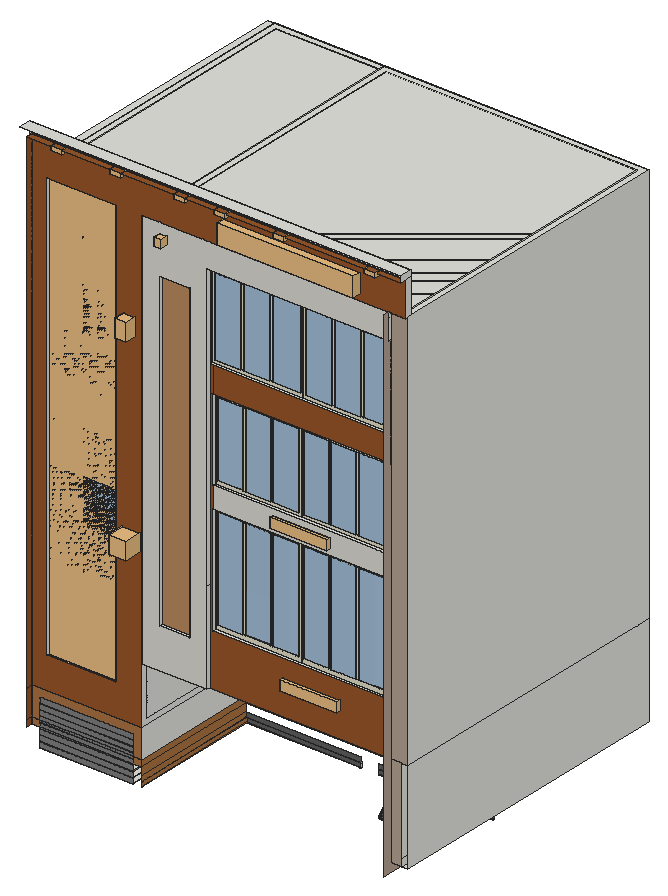
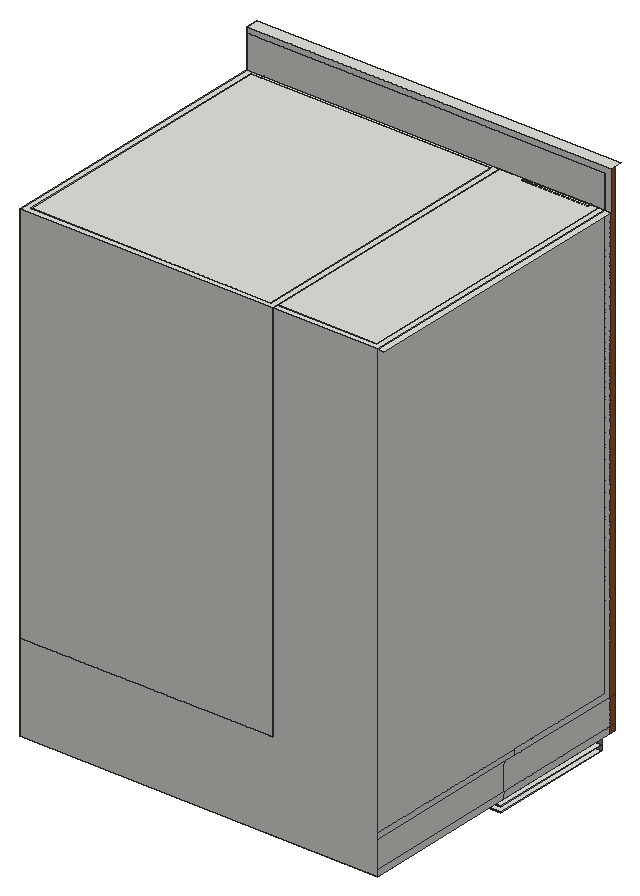
# SketchUp Ruby script. Lengths in inches.
U = 1.inch
M = Sketchup.active_model
def pt(a) = Geom::Point3d.new(a.map { |v| v * U })
def face(e, loops, mat)
  f = e.add_face(loops[0].map { |a| pt(a) })
  loops[1..].each { |l| e.add_face(l.map { |a| pt(a) }).erase! }
  f.material = f.back_material = mat if mat
  f
end
# faces: each face lists its corners as indices into pts; further lists are holes
def faces(e, pts, list, mat = nil) = list.each { |f| face(e, (f[0].is_a?(Array) ? f : [f]).map { |l| l.map { |i| pts[i] } }, mat) }
# xy, xz, yz: faces in a plane at the given z, y or x. An outline is a flat list of corners, or four numbers for a rectangle; further outlines are holes
def ring(l) = l.size == 4 ? [[l[0], l[1]], [l[2], l[1]], [l[2], l[3]], [l[0], l[3]]] : l.each_slice(2).to_a
def flat(e, list, mat, &to3) = list.each { |f| face(e, (f[0].is_a?(Array) ? f : [f]).map { |l| ring(l).map { |u, v| to3.(u, v) } }, mat) }
def xy(e, z, list, mat = nil) = flat(e, list, mat) { |x, y| [x, y, z] }
def xz(e, y, list, mat = nil) = flat(e, list, mat) { |x, z| [x, y, z] }
def yz(e, x, list, mat = nil) = flat(e, list, mat) { |y, z| [x, y, z] }
def lines(e, pts, list) = list.each { |a, b| e.add_line(pt(pts[a]), pt(pts[b])) }
# prism: a flat outline (further loops are holes) pulled along v
def prism(e, loops, v, mat = nil)
  f = face(e, loops, mat); d = Geom::Vector3d.new(v.map { |x| x * U })
  f.pushpull(f.normal.samedirection?(d) ? d.length : -d.length)
end
def box(e, o, s, mat = nil) = prism(e, [[o, [o[0] + s[0], o[1], o[2]], [o[0] + s[0], o[1] + s[1], o[2]], [o[0], o[1] + s[1], o[2]]]], [0, 0, s[2]], mat)
def at(x, y, z, deg = 0) = Geom::Transformation.translation(pt([x, y, z])) * Geom::Transformation.rotation(ORIGIN, Z_AXIS, deg.degrees)
def axes(o, x, y, z) = Geom::Transformation.new([*x, 0, *y, 0, *z, 0, *pt(o).to_a, 1])
def part(name) = M.definitions.add(name)
# library, detail: a bought-in or finely detailed component or shape, given as its bounding box
def library(name, o, s) = part(name).tap { |d| box(d.entities, o, s) }
def detail(e, o, s) = box(e.add_group.entities, o, s)
def put(e, d, t, mat = nil) = e.add_instance(d, t).tap { |i| i.material = mat if mat }
def group(e, t, mat = nil) = e.add_group.tap { |g| g.transformation = t; g.material = mat if mat }.entities
root = M.entities
M.materials.add("Glass").color = [171, 209, 242]
M.materials["Glass"].alpha = 0.09
M.materials.add("Plastic_SSS_01_White").color = [225, 221, 201]
M.materials.add("[0020_Red]").color = [234, 0, 0]
M.materials.add("[0098_DodgerBlue]").color = [162, 189, 214]
M.materials.add("[0133_Gray]").color = [96, 96, 96]
M.materials.add("[0133_Gray]1").color = [128, 128, 128]
M.materials.add("[0135_DarkGray]").color = [81, 81, 81]
M.materials.add("[Formica Speckled Grey]").color = [94, 105, 111]
M.materials.add("[Roofing Scalloped]").color = [186, 138, 96]
M.materials.add("[Terrazzo Tile Light]").color = [219, 217, 210]
M.materials.add("[Travertine Small Tile]").color = [180, 162, 145]
M.materials.add("[Wood Cherry Original]").color = [152, 86, 42]
M.materials.add("[Wood Floor]").color = [172, 116, 67]
c1 = part("Glass Door - Open Shower")
box(c1.entities,[0,0,0.95],[40,1.5,72])
c2 = library("Group\#2",[0,0,0],[96.3125,10,597])
c3 = library("SIGNAGE",[0.49,0,0],[52.61,9.87,1])
c4 = part("Window frame")
xy(c4.entities,0,[[[104.47,83.98,176.47,131.98],[106.47,85.98,174.47,129.98]],[127.47,85.98,129.47,129.98],[150.47,85.98,152.47,129.98]],"Plastic_SSS_01_White")
xy(c4.entities,2,[[[104.47,83.98,176.47,131.98],[106.47,85.98,174.47,129.98]],[127.47,85.98,129.47,129.98],[150.47,85.98,152.47,129.98]],"Plastic_SSS_01_White")
xz(c4.entities,83.98,[[104.47,0,176.47,2]],"Plastic_SSS_01_White")
xz(c4.entities,85.98,[[106.47,0,127.47,2],[127.47,0,129.47,2],[129.47,0,150.47,2],[150.47,0,152.47,2],[152.47,0,174.47,2]],"Plastic_SSS_01_White")
xz(c4.entities,129.98,[[106.47,0,127.47,2],[127.47,0,129.47,2],[129.47,0,150.47,2],[150.47,0,152.47,2],[152.47,0,174.47,2]],"Plastic_SSS_01_White")
xz(c4.entities,131.98,[[104.47,0,176.47,2]],"Plastic_SSS_01_White")
yz(c4.entities,104.47,[[83.98,0,131.98,2]],"Plastic_SSS_01_White")
yz(c4.entities,106.47,[[85.98,0,129.98,2]],"Plastic_SSS_01_White")
yz(c4.entities,127.47,[[85.98,0,129.98,2]],"Plastic_SSS_01_White")
yz(c4.entities,129.47,[[85.98,0,129.98,2]],"Plastic_SSS_01_White")
yz(c4.entities,150.47,[[85.98,0,129.98,2]],"Plastic_SSS_01_White")
yz(c4.entities,152.47,[[85.98,0,129.98,2]],"Plastic_SSS_01_White")
yz(c4.entities,174.47,[[85.98,0,129.98,2]],"Plastic_SSS_01_White")
yz(c4.entities,176.47,[[83.98,0,131.98,2]],"Plastic_SSS_01_White")
c5 = part("Window pane")
box(c5.entities,[0,0,0],[67.88,44,0.5])
c6 = part("Glazed window unit")
put(c6.entities,c4,at(-104.47,-83.98,0))
put(c6.entities,c5,at(2,2,0.7),"Glass")
c7 = part("window")
p = [[-596.28,88.12,20.39],[-668.28,88.12,20.39]]
lines(c7.entities,p,[[0,1]])
put(c7.entities,c6,axes([-668.28,88.12,20.39],[1,0,0],[0,0,1],[0,-1,0]))
c8 = library("Omni Light\#3",[-12,-12,-12],[24,24,24])
c9 = library("Omni Light\#2",[-12,-12,-12],[24,24,24])
c10 = library("Spot Light",[-5.1,-5.1,-11.05],[10.2,10.2,11.05])
c11 = library("Building Name",[0.96,0,0],[81.96,12.64,1])
c12 = library("Omni Light\#4",[-12,-12,-12],[24,24,24])
xy(root,93.95,[[21,9,150.5,192.6875]])
xy(root,94.45,[[21,9,150.5,192.6875]])
xy(root,94.7,[[347,191.6875,507.47,192.6875],[162.5,192.0625,322.97,192.6875]])
xy(root,95.2,[[347,191.6875,507.47,192.6875],[162.5,192.0625,322.97,192.6875]])
xy(root,101.1,[[346.99,191.6875,507.46,192.6875],[162.5,192.0625,322.97,192.6875]])
xy(root,101.6,[[162.5,191.6875,322.97,192.6875],[346.99,191.6875,507.45,192.6875]])
xy(root,101.82,[[21,9,150.5,192.6875]])
xy(root,102.32,[[21,9,150.5,192.6875]])
xy(root,102.5,[[[404.69,160.97,507.9,164.35,506.48,179.71,403.27,176.33],[414.3,165.74,413.36,165.77,412.49,165.95,411.73,166.27,411.15,166.72,410.78,167.26,410.65,167.86,410.76,168.47,411.12,169.06,411.69,169.57,412.43,169.99,413.3,170.28,414.23,170.41,415.17,170.39,416.04,170.21,416.8,169.88,417.38,169.43,417.75,168.89,417.88,168.29,417.77,167.68,417.41,167.1,416.85,166.58,416.1,166.17,415.23,165.88]],[414.3,165.74,415.23,165.88,416.1,166.17,416.85,166.58,417.41,167.1,417.77,167.68,417.88,168.29,417.75,168.89,417.38,169.43,416.8,169.88,416.04,170.21,415.17,170.39,414.23,170.41,413.3,170.28,412.43,169.99,411.69,169.57,411.12,169.06,410.76,168.47,410.65,167.86,410.78,167.26,411.15,166.72,411.73,166.27,412.49,165.95,413.36,165.77],[403.27,176.33,401.86,191.6875,505.0625,195.07,506.48,179.71]],"[Formica Speckled Grey]")
xy(root,109.69,[[21,9,150.5,192.6875]])
xy(root,110.19,[[21,9,150.5,192.6875]])
xy(root,117.14,[[[403.27,176.33,506.48,179.71,505.0625,195.07,401.86,191.6875],[412.3,181.1,412.125,181.12,411.95,181.125,411.67,181.18,411.39,181.22,411.24,181.27,411.07,181.31,410.84,181.41,410.59,181.49,410.46,181.57,410.32,181.63,410.14,181.77,409.93,181.9,409.85,182,409.74,182.08,409.62,182.25,409.48,182.41,409.4375,182.52,409.37,182.625,409.33,182.81,409.26,182.99,409.26,183.11,409.23,183.22,409.27,183.41,409.28,183.6,409.33,183.71,409.35,183.83,409.46,184.01,409.54,184.2,409.63,184.3,409.7,184.42,409.88,184.58,410.03,184.75,410.16,184.83,410.27,184.93,410.5,185.0625,410.71,185.2,410.87,185.27,411.01,185.35,411.28,185.4375,411.54,185.54,411.72,185.58,411.88,185.63,412.17,185.68,412.46,185.74,412.64,185.74,412.82,185.77,413.11,185.76,413.4,185.77,413.57,185.75,413.75,185.75,414.03,185.69,414.31,185.65,414.46,185.6,414.63,185.57,414.86,185.46,415.11,185.38,415.24,185.3,415.38,185.24,415.5625,185.1,415.77,184.97,415.85,184.88,415.96,184.79,416.08,184.625,416.22,184.46,416.26,184.35,416.33,184.25,416.375,184.06,416.44,183.88,416.44,183.77,416.47,183.65,416.43,183.46,416.42,183.27,416.375,183.16,416.35,183.04,416.24,182.86,416.16,182.67,416.07,182.57,416,182.46,415.82,182.3,415.67,182.125,415.54,182.04,415.43,181.94,415.2,181.8125,414.99,181.67,414.83,181.6,414.6875,181.52,414.42,181.4375,414.16,181.33,413.98,181.29,413.82,181.24,413.53,181.2,413.24,181.14,413.0625,181.13,412.88,181.1,412.59,181.11]],[412.88,181.1,413.0625,181.13,412.59,181.11],[412.125,181.12,411.67,181.18,411.95,181.125],[413.53,181.2,413.82,181.24,413.98,181.29],[411.24,181.27,410.84,181.41,411.07,181.31],
  [414.42,181.4375,414.6875,181.52,414.83,181.6],[410.46,181.57,410.14,181.77,410.32,181.63],[415.2,181.8125,415.43,181.94,415.54,182.04],[409.85,182,409.62,182.25,409.74,182.08],[415.82,182.3,416,182.46,416.07,182.57],
  [409.4375,182.52,409.33,182.81,409.37,182.625],[416.24,182.86,416.35,183.04,416.375,183.16],[409.26,183.11,409.27,183.41,409.23,183.22],[416.43,183.46,416.47,183.65,416.44,183.77],[409.33,183.71,409.46,184.01,409.35,183.83],
  [416.375,184.06,416.33,184.25,416.26,184.35],[409.63,184.3,409.88,184.58,409.7,184.42],[416.08,184.625,415.96,184.79,415.85,184.88],[410.16,184.83,410.5,185.0625,410.27,184.93],[415.5625,185.1,415.38,185.24,415.24,185.3],
  [410.87,185.27,411.28,185.4375,411.01,185.35],[414.86,185.46,414.63,185.57,414.46,185.6],[411.72,185.58,412.17,185.68,411.88,185.63],[414.03,185.69,413.75,185.75,413.57,185.75],[412.64,185.74,413.11,185.76,412.82,185.77]],"[Formica Speckled Grey]")
xy(root,117.5625,[[21,9,150.5,192.6875]])
xy(root,118.0625,[[21,9,150.5,192.6875]])
xy(root,120,[[9,9,9,201.6875,18,201.6875,18,423.6875,522.4375,423.6875,522.4375,201.6875,162.5,201.6875,162.5,9],[522.4375,13,522.4375,191.6875,162.5,191.6875,162.5,201.6875,522.4375,201.6875,522.4375,423.6875,18,423.6875,18,201.6875,9,201.6875,9,432.6875,531.4375,432.6875,531.4375,13]])
xy(root,120,[[507.4375,13,522.4375,191.6875]],"[Travertine Small Tile]")
xy(root,125.43,[[21,191.6875,150.5,192.6875]])
xy(root,125.43,[[21,9,150.5,191.6875]],"[0133_Gray]1")
xy(root,125.93,[[21,191.6875,150.5,192.6875]])
xy(root,125.93,[[21,9,150.5,191.6875]],"[0133_Gray]1")
xy(root,129,[[9,9,162.5,9,162.5,423.6875,18,423.6875,18,201.6875,9,201.6875],[162.5,191.6875,507.4375,215.6875],[507.4375,191.6875,522.4375,215.6875],[186.5,215.6875,504.4375,215.6875,504.4375,224.6875,522.4375,224.6875,522.4375,423.6875,186.5,423.6875]])
xy(root,133.3,[[21,9,150.5,192.6875]])
xy(root,133.8,[[21,9,150.5,192.6875]])
xy(root,141.18,[[21,9,150.5,192.6875]])
xy(root,141.68,[[21,9,150.5,192.6875]])
xy(root,149.05,[[21,9,150.5,192.6875]])
xy(root,149.55,[[21,9,150.5,192.6875]])
xy(root,168,[[18,9,162.5,201.6875],[9,181.6875,18,201.6875]])
xy(root,168,[[9,9,18,181.6875]],"[Wood Floor]")
xy(root,177,[[9,18,18,181.6875],[18,18,162.5,201.6875]])
xy(root,213,[[30.5,9,126,18]])
xy(root,232,[[186.5,215.6875,504.4375,224.6875]])
xy(root,249,[[162.5,9,162.5,215.6875,522.4375,215.6875,522.4375,13,254.07,13,254.07,9],[522.4375,13,531.4375,432.6875],[162.5,215.6875,162.5,432.6875,522.4375,432.6875,522.4375,423.6875,186.5,423.6875,186.5,224.6875,522.4375,224.6875,522.4375,215.6875],[186.5,224.6875,522.4375,423.6875]])
xy(root,258,[[171.5,22,522.4375,423.6875]])
xy(root,305.18,[[187.89,9,230.08,13]])
xy(root,322.125,[[259.07,13,498.4375,22]])
xy(root,474,[[259.07,13,498.4375,22]])
xy(root,504,[[259.07,13,498.4375,22]])
xy(root,618,[[259.07,13,498.4375,22],[498.4375,13,507.4375,22]])
xy(root,654,[[254.07,13,507.4375,22]])
xy(root,742.06,[[187.89,9,230.08,13]])
xy(root,774,[[254.07,9,507.4375,13],[254.07,13,507.4375,22]])
xy(root,810,[[30.5,9,30.5,18,126.5,18,126,9],[126,9,126.5,18,162.5,18,162.5,9],[162.5,9,507.4375,18],[507.4375,9,531.4375,13],[507.4375,13,507.4375,22,522.4375,22,522.4375,423.6875,171.5,423.6875,171.5,22,507.4375,22,507.4375,18,531.4375,18,531.4375,13],
  [507.4375,13,531.4375,18],[0,18,9,432.6875],[9,18,18,18,18,423.6875,162.5,423.6875,162.5,432.6875,9,432.6875],[18,18,162.5,423.6875],[162.5,18,531.4375,432.6875]])
xy(root,858,[[9,9,531.4375,18]])
xy(root,858,[[9,0,531.4375,9]],"[Wood Cherry Original]")
xy(root,866.75,[[0,0,531.4375,18]])
xz(root,9,[[21,94.45,150.5,101.82],[21,102.32,150.5,109.69],[21,110.19,150.5,117.5625],[21,118.0625,150.5,120],[21,120,150.5,125.43],
  [21,125.93,150.5,129],[21,129,150.5,133.3],[21,133.8,150.5,141.18],[21,141.68,150.5,149.05],[21,149.55,150.5,157.42]],"[0133_Gray]1")
xz(root,9,[[[162.5,249,254.07,249,254.07,774,507.4375,774,507.4375,810,162.5,810],[187.89,305.18,230.08,742.06]]],"[Terrazzo Tile Light]")
xz(root,9,[[9,168,162.5,168,162.5,810,126,810,126,213,30.5,213,30.5,810,531.4375,810,531.4375,858,9,858]],"[Wood Cherry Original]")
xz(root,9,[[9,120,21,129],[150.5,120,162.5,129],[9,129,21,129,21,157.42,150.5,157.42,150.5,129,162.5,129,162.5,168,9,168]],"[Wood Floor]")
xz(root,13,[[78.1,630.9,78.18,690.1],[78.1,690.54,124.85,690.6,78.1,690.6]])
xz(root,13,[[30.76,332.4,78.59,392.1],[78.59,332.4,125.26,392.1],[30.76,392.1,78.43,451.3],[78.43,392.1,125.18,451.3],[78.34,451.3,125.18,511],
  [30.68,451.8,77.84,511],[30.43,511.5,77.84,571.2],[78.34,511.5,125.01,571.2],[30.43,571.2,77.76,630.4],[78.26,571.2,124.93,630.4],
  [30.5,630.9,78.1,690.1],[78.18,630.9,124.93,630.9,124.93,690.6,124.85,690.6,78.1,690.54,78.1,690.1,78.18,690.1],[30.5,690.6,77.6,749.8],[78.1,690.6,124.85,690.6,124.77,750.36,78.02,750.3],[30.5,750.3,77.9375,809.5],
  [78.02,750.3,124.77,750.36,124.6875,809.5,77.9375,809.4375]],"[0098_DodgerBlue]")
xz(root,13,[[187.89,305.18,230.08,742.06]],"[Roofing Scalloped]")
xz(root,13,[[259.07,474,498.4375,504]],"[Terrazzo Tile Light]")
xz(root,13,[[507.4375,120,522.4375,249],[507.4375,249,531.4375,810]],"[Travertine Small Tile]")
xz(root,13,[[254.07,249,507.4375,249,507.4375,618,498.4375,618,498.4375,322.125,259.07,322.125,259.07,618,254.07,618],[254.07,618,259.07,654],[259.07,618,498.4375,654],[498.4375,618,507.4375,654]],"[Wood Cherry Original]")
xz(root,13.5,[[31,213.5,78.25,213.5625,78.17,272.2,30.92,272.14],[78.67,213.5,125.5,272.2],[30.92,272.7,78.67,272.76,78.59,331.9,30.84,331.84],[78.67,272.7,125.34,331.9]],"[0098_DodgerBlue]")
xz(root,17.5,[[262.4,328.54,297.31,469.78],[382.08,328.54,416.99,469.78],[420.3125,328.54,455.22,469.78],[300.63,508.75,335.54,613.25],[338.86,508.75,375.43,613.25],
  [382.08,508.75,416.99,613.25],[420.3125,508.75,455.22,613.25],[458.54,508.75,495.11,613.25],[257.6,658.94,294.67,767.62],[298.19,658.94,335.26,767.62],
  [338.79,658.94,377.61,767.62],[384.67,658.94,421.73,767.62],[425.26,658.94,462.33,767.62]],"[0098_DodgerBlue]")
xz(root,18,[[18,177,18,810,30.5,810,30.5,213,126,213,126.5,810,162.5,810,162.5,177],[30.5,213,30.5,810,126.5,810,126,213],[0,810,0,866.75,531.4375,866.75,531.4375,858,9,858,9,810],[9,810,531.4375,858]])
xz(root,22,[[[171.5,258,171.5,810,507.4375,810,507.4375,774,254.07,774,254.07,654,507.4375,654,507.4375,618,259.07,618,259.07,504,498.4375,504,498.4375,618,507.4375,618,507.4375,258],[259.07,322.125,498.4375,474]],[507.4375,258,522.4375,810]])
xz(root,181.6875,[[9,168,18,177]])
xz(root,191.6875,[[162.5,120,507.4375,129],[507.4375,120,522.4375,129],[21,125.43,150.5,125.93]])
xz(root,191.6875,[[347,95.2,507.47,95.2,507.46,101.1,346.99,101.1],[162.5,101.6,322.97,108],[346.99,101.6,507.45,101.6,507.4375,108,346.97,108]],"[0133_Gray]")
xz(root,192.0625,[[162.5,95.2,322.97,101.1]],"[0133_Gray]")
xz(root,192.6875,[[347,94.7,507.47,95.2],[346.99,101.1,507.46,101.1,507.45,101.6,346.99,101.6]])
xz(root,192.6875,[[21,93.95,150.5,94.45],[162.5,94.7,322.97,95.2],[162.5,101.1,322.97,101.6],[21,101.82,150.5,102.32],[21,109.69,150.5,110.19],
  [21,117.5625,150.5,118.0625],[21,125.43,150.5,125.93],[21,133.3,150.5,133.8],[21,141.18,150.5,141.68],[21,149.05,150.5,149.55]],"[0135_DarkGray]")
xz(root,201.6875,[[9,120,18,129],[9,129,18,168],[18,168,162.5,177]])
xz(root,215.6875,[[162.5,129,186.5,129,186.5,232,504.4375,232,504.4375,129,522.4375,129,522.4375,249,162.5,249]],"[0133_Gray]")
xz(root,224.6875,[[504.4375,129,504.4375,232,186.5,232,186.5,249,522.4375,249,522.4375,129]])
xz(root,423.6875,[[18,129,162.5,810],[186.5,129,522.4375,249],[171.5,258,522.4375,810]])
xz(root,432.6875,[[9,120,9,810,162.5,810,162.5,249,531.4375,249,531.4375,120],[162.5,249,531.4375,810]])
yz(root,9,[[9,120,201.6875,129],[201.6875,120,432.6875,129],[9,129,201.6875,168],[201.6875,129,432.6875,168],[9,168,9,858,18,858,18,177,181.6875,177,181.6875,168],
  [181.6875,168,432.6875,177],[18,177,432.6875,810]])
yz(root,9,[[0,120,9,129],[0,129,9,168],[0,168,9,858]],"[Wood Cherry Original]")
yz(root,18,[[201.6875,129,423.6875,129,423.6875,810,18,810,18,177,201.6875,177],[181.6875,168,201.6875,177]])
yz(root,21,[[9,93.95,192.6875,94.45],[9,101.82,192.6875,102.32],[9,109.69,192.6875,110.19],[9,117.5625,192.6875,118.0625],[191.6875,125.43,192.6875,125.93],
  [9,133.3,192.6875,133.8],[9,141.18,192.6875,141.68],[9,149.05,192.6875,149.55]])
yz(root,21,[[9,125.43,191.6875,125.93]],"[Wood Floor]")
yz(root,30.5,[[9,213,18,810]])
yz(root,150.5,[[191.6875,125.43,192.6875,125.93],[9,133.3,192.6875,133.8],[9,141.18,192.6875,141.68],[9,149.05,192.6875,149.55]])
yz(root,150.5,[[9,93.95,192.6875,94.45],[9,101.82,192.6875,102.32],[9,109.69,192.6875,110.19],[9,117.5625,192.6875,118.0625],[9,125.43,191.6875,125.93]],"[Wood Floor]")
yz(root,162.5,[[191.6875,120,201.6875,129],[9,129,201.6875,168],[201.6875,129,215.6875,177],[215.6875,129,423.6875,249],[9,168,201.6875,168,201.6875,177,18,177,18,249,9,249],
  [18,177,215.6875,249],[9,249,18,810],[18,249,423.6875,810],[423.6875,249,432.6875,810]])
yz(root,162.5,[[9,94.7,192.6875,95.2],[9,95.2,192.0625,101.1],[9,101.1,192.6875,101.6],[9,101.6,191.6875,108],[9,108,191.6875,120],
  [9,120,191.6875,129]],"[Wood Floor]")
yz(root,171.5,[[22,258,423.6875,810]])
yz(root,186.5,[[215.6875,129,423.6875,129,423.6875,249,224.6875,249,224.6875,232,215.6875,232]])
yz(root,187.89,[[9,305.18,13,742.06]])
yz(root,230.08,[[9,305.18,13,742.06]])
yz(root,254.07,[[9,249,13,378],[9,378,13,774],[13,654,22,774]])
yz(root,259.07,[[13,322.125,22,474],[13,504,22,618]])
yz(root,322.97,[[191.6875,94.7,192.6875,95.2],[191.6875,95.2,192.0625,101.1],[191.6875,101.1,192.6875,101.6]])
yz(root,346.99,[[191.6875,101.1,192.6875,101.6]])
yz(root,347,[[191.6875,94.7,192.6875,95.2]])
yz(root,498.4375,[[13,322.125,22,474],[13,504,22,618]])
yz(root,504.4375,[[215.6875,129,224.6875,232]])
yz(root,507.4375,[[13,618,22,654],[13,654,22,774],[9,774,13,810],[13,774,22,810]])
yz(root,507.4375,[[0.125,108,0.125,810,9,810,9,774,13,774,13,120,191.6875,120,191.6875,108]],"[Travertine Small Tile]")
yz(root,522.4375,[[13,120,191.6875,129],[13,129,215.6875,249],[215.6875,129,224.6875,249],[224.6875,129,423.6875,249],[22,258,423.6875,810]])
yz(root,531.4375,[[13,120,432.6875,249],[13,249,432.6875,810],[9,810,18,858],[0,858,18,866.75]])
p = [[416.78,122.77,113.62],[416.68,123.91,114.71],[417.55,124.2,114.47],[417.66,122.95,113.27],[418.96,108.84,99.82],[418.09,108.56,100.06],
  [418.48,124.34,114.41],[418.6,123.05,113.1875],[419.9,108.98,99.77],[419.42,124.3125,114.54],[419.53,123.09,113.375],[420.83,108.95,99.9],
  [420.29,124.13,114.84],[420.39,123.05,113.82],[421.71,108.77,100.2],[416.02,122.55,114.21],[415.93,123.5,115.11],[417.35,108.14,100.47],
  [421.05,123.8,115.31],[421.125,122.94,114.49],[422.46,108.45,100.66],[415.43,122.28,114.99],[415.37,122.98,115.66],[416.78,107.62,101.01],
  [421.63,123.36,115.89],[421.68,122.77,115.34],[423.04,108,101.25],[415.05,122,115.93],[415.01,122.4,116.3],[416.43,107.04,101.66],
  [422,122.81,116.57],[422.02,122.55,116.31],[423.41,107.46,101.92],[414.9,121.72,116.94],[414.9,121.78,117],[416.3125,106.43,102.36],
  [422.13,122.22,117.28],[423.54,106.92,102.69],[423.55,106.86,102.63],[416.42,106.1,103.33],[415.03,121.1875,117.71],[416.45,105.83,103.07],
  [413.36,165.77,102.5],[414.3,165.74,102.5],[414.3,165.74,163.8],[413.36,165.77,163.67],[415.23,165.88,102.5],[415.23,165.88,163.74],
  [412.49,165.95,102.5],[412.49,165.95,163.36],[411.73,166.27,102.5],[411.73,166.27,162.9],[416.1,166.17,102.5],[416.1,166.17,163.5],
  [416.85,166.58,102.5],[416.85,166.58,163.09],[411.15,166.72,102.5],[411.15,166.72,162.31],[417.41,167.1,102.5],[417.41,167.1,162.55],
  [410.78,167.26,102.5],[410.78,167.26,161.64],[417.77,167.68,102.5],[417.77,167.68,161.91],[410.65,167.86,102.5],[410.65,167.86,160.93],
  [417.88,168.29,102.5],[417.88,168.29,161.2],[410.76,168.47,102.5],[410.76,168.47,160.23],[417.75,168.89,102.5],[417.75,168.89,160.49],
  [411.12,169.06,102.5],[411.12,169.06,159.58],[417.38,169.43,102.5],[417.38,169.43,159.82],[411.69,169.57,102.5],[411.69,169.57,159.04],
  [416.8,169.88,102.5],[416.8,169.88,159.23],[412.43,169.99,102.5],[412.43,169.99,158.63],[416.04,170.21,102.5],[416.04,170.21,158.77],
  [413.3,170.28,102.5],[413.3,170.28,158.39],[415.17,170.39,102.5],[415.17,170.39,158.47],[414.23,170.41,102.5],[414.23,170.41,158.34],
  [401.86,191.6875,102.5],[403.27,176.33,102.5],[403.27,176.33,117.14],[401.86,191.6875,117.14],[506.48,179.71,102.5],[506.48,179.71,117.14],
  [505.0625,195.07,102.5],[505.0625,195.07,117.14],[422.02,121.61,117.98],[423.4,106.64,103.71],[423.43,106.25,103.34],[416.76,105.875,104.3],
  [415.4,120.65,118.39],[416.82,105.29,103.74],[421.66,121.02,118.625],[423.01,106.36,104.64],[423.08,105.66,103.98],[417.32,105.7,105.15],
  [415.98,120.2,118.97],[417.4,104.84,104.33],[421.09,120.5,119.17],[422.42,106.1,105.43],[422.51,105.15,104.52],[418.05,105.59,105.82],
  [416.74,119.87,119.4375],[418.15,104.51,104.79],[420.35,120.09,119.57],[421.66,105.87,106.02],[421.77,104.73,104.93],[418.91,105.55,106.26],
  [417.61,119.69,119.74],[419.03,104.33,105.1],[419.48,119.8,119.8125],[420.78,105.7,106.37],[420.9,104.44,105.17],[419.85,105.59,106.45],
  [418.55,119.67,119.87],[419.96,104.31,105.23],[416.25,138.3,127.91],[416.13,139.56,129.11],[417.0625,139.69,129.05],[417.18,138.41,127.83],
  [418,139.67,129.18],[418.11,138.45,128.02],[415.37,138.13,128.26],[415.26,139.27,129.35],[418.875,139.49,129.49],[418.98,138.41,128.46],
  [414.61,137.91,128.85],[414.52,138.86,129.76],[419.63,139.16,129.95],[419.71,138.3,129.13],[414.01,137.64,129.64],[413.95,138.34,130.3],
  [420.21,138.71,130.54],[420.27,138.13,129.98],[413.63,137.36,130.57],[413.6,137.75,130.94],[420.58,138.17,131.21],[420.61,137.9,130.95],
  [413.49,137.08,131.59],[413.48,137.14,131.65],[420.71,137.58,131.92],[422.125,122.28,117.34],[415.01,121.46,117.97],[413.61,136.55,132.36],
  [412.3,181.1,168.71],[411.39,181.22,169.34],[411.39,181.22,117.14],[411.67,181.18,117.14],[412.125,181.12,117.14],[412.3,181.1,117.14],
  [413.24,181.14,168.5625],[412.59,181.11,117.14],[413.0625,181.13,117.14],[413.24,181.14,117.14],[414.16,181.33,168.9],[413.53,181.2,117.14],
  [413.98,181.29,117.14],[414.16,181.33,117.14],[410.59,181.49,170.4],[410.59,181.49,117.14],[410.84,181.41,117.14],[411.24,181.27,117.14],
  [414.99,181.67,169.7],[414.42,181.4375,117.14],[414.83,181.6,117.14],[414.99,181.67,117.14],[409.93,181.9,171.83],[409.93,181.9,117.14],
  [410.14,181.77,117.14],[410.46,181.57,117.14],[415.67,182.125,170.91],[415.2,181.8125,117.14],[415.54,182.04,117.14],[415.67,182.125,117.14],
  [409.48,182.41,173.52],[409.48,182.41,117.14],[409.62,182.25,117.14],[409.85,182,117.14],[416.16,182.67,172.45],[415.82,182.3,117.14],
  [416.07,182.57,117.14],[416.16,182.67,117.14],[409.26,182.99,175.35],[409.26,182.99,117.14],[409.33,182.81,117.14],[409.4375,182.52,117.14],
  [416.42,183.27,174.2],[416.24,182.86,117.14],[416.375,183.16,117.14],[416.42,183.27,117.14],[409.28,183.6,177.22],[409.28,183.6,117.14],
  [409.27,183.41,117.14],[409.26,183.11,117.14],[416.44,183.88,176.07],[416.43,183.46,117.14],[416.44,183.77,117.14],[416.44,183.88,117.14],
  [409.54,184.2,178.97],[409.54,184.2,117.14],[409.46,184.01,117.14],[409.33,183.71,117.14],[416.22,184.46,177.9],[416.375,184.06,117.14],
  [416.26,184.35,117.14],[416.22,184.46,117.14],[410.03,184.75,180.51],[410.03,184.75,117.14],[409.88,184.58,117.14],[409.63,184.3,117.14],
  [415.77,184.97,179.59],[416.08,184.625,117.14],[415.85,184.88,117.14],[415.77,184.97,117.14],[410.71,185.2,181.72],[410.71,185.2,117.14],
  [410.5,185.0625,117.14],[410.16,184.83,117.14],[415.11,185.38,181.02],[415.5625,185.1,117.14],[415.24,185.3,117.14],[415.11,185.38,117.14],
  [411.54,185.54,182.52],[411.54,185.54,117.14],[411.28,185.4375,117.14],[410.87,185.27,117.14],[414.31,185.65,182.08],[414.86,185.46,117.14],
  [414.46,185.6,117.14],[414.31,185.65,117.14],[412.46,185.74,182.86],[412.46,185.74,117.14],[412.17,185.68,117.14],[411.72,185.58,117.14],
  [413.4,185.77,182.71],[413.4,185.77,117.14],[413.11,185.76,117.14],[412.64,185.74,117.14],[414.03,185.69,117.14],[413.57,185.75,117.14],
  [420.6,136.97,132.62],[421.98,122,118.35],[415.35,121.23,118.94],[413.98,136.01,133.03],[420.25,136.38,133.27],[421.6,121.72,119.29],
  [415.9,121.06,119.79],[414.56,135.56,133.62],[419.68,135.86,133.81],[421.01,121.46,120.07],[416.64,120.95,120.46],[415.32,135.23,134.08],
  [418.93,135.45,134.22],[420.25,121.23,120.66],[417.5,120.91,120.91],[416.19,135.05,134.38],[418.07,135.16,134.46],[419.37,121.06,121.01],
  [418.43,120.95,121.09],[417.13,135.03,134.51],[413.85,154.63,143.99],[414.71,154.92,143.75],[414.83,153.66,142.56],[413.95,153.49,142.9],
  [415.65,155.05,143.69],[415.77,153.77,142.47],[416.59,155.03,143.82],[416.7,153.81,142.66],[417.46,154.85,144.13],[417.56,153.77,143.1],
  [413.1,154.22,144.4],[413.1875,153.27,143.49],[418.22,154.52,144.59],[418.29,153.66,143.77],[412.6,153,144.28],[412.53,153.7,144.94],
  [418.8,154.07,145.18],[418.85,153.49,144.62],[412.22,152.72,145.21],[412.18,153.11,145.59],[419.17,153.53,145.85],[419.19,153.26,145.59],
  [412.07,152.4375,146.23],[412.07,152.5,146.29],[419.3,152.9375,146.5625],[420.71,137.64,131.98],[413.59,136.82,132.61],[412.2,151.91,147],
  [419.18,152.32,147.26],[420.5625,137.36,133],[413.93,136.59,133.59],[412.57,151.36,147.67],[418.83,151.74,147.91],[420.18,137.08,133.93],
  [414.49,136.42,134.4375],[413.15,150.92,148.26],[418.26,151.22,148.45],[419.59,136.8125,134.72],[415.22,136.31,135.11],[413.9,150.59,148.72],
  [417.52,150.81,148.86],[418.83,136.59,135.3],[416.08,136.27,135.55],[414.78,150.41,149.03],[416.65,150.52,149.1],[417.95,136.42,135.65],
  [417.01,136.31,135.73],[415.72,150.39,149.16],[413.41,169.02,157.2],[414.35,169.13,157.12],[415.28,169.17,157.3],[412.53,168.85,157.55],
  [416.14,169.13,157.74],[411.77,168.625,158.13],[416.88,169.02,158.41],[411.18,168.36,158.92],[417.43,168.85,159.26],[410.8,168.08,159.85],
  [417.77,168.62,160.24],[410.66,167.8,160.87],[419.29,153,146.62],[412.17,152.18,147.26],[419.15,152.72,147.64],[412.51,151.95,148.23],
  [418.77,152.4375,148.57],[413.07,151.78,149.08],[418.17,152.17,149.36],[413.8,151.67,149.75],[417.41,151.95,149.95],[414.67,151.63,150.19],
  [416.53,151.77,150.29],[415.6,151.67,150.375],[417.875,168.36,161.26],[410.76,167.53,161.9],[417.73,168.08,162.28],[411.1,167.31,162.87],
  [417.35,167.79,163.21],[411.65,167.14,163.72],[416.76,167.53,164],[412.39,167.03,164.39],[416,167.31,164.59],[413.25,166.99,164.83],
  [415.12,167.13,164.94],[414.18,167.03,165.02],[126,9,810],[126.5,18,810],[126,9,213],[126,18,213],
  [336.03,17.5,469.78],[300.63,17.5,469.78],[300.63,18.8,328.55],[336.03,18.8,328.55],[338.86,17.5,469.78],[338.86,17.5,328.55],
  [375.23,18.8,328.55],[375.23,18.8,469.78],[494.91,18.8,328.55],[494.91,18.8,469.78],[458.54,17.5,469.78],[458.54,17.5,328.55],
  [78.51,14,392.1],[125.18,13,392.1],[125.18,13,451.3],[78.51,14,451.3],[262.4,17.5,508.75],[297.45,19.27,508.75],
  [297.45,19.27,613.25],[262.4,17.5,613.25],[465.86,17.5,767.62],[465.86,17.5,658.94],[504.47,20.09,658.94],[504.47,20.09,767.62]]
faces(root,p,[[0,1,2,3,4,5],[3,2,6,7,8,4],[7,6,9,10,11,8],[10,9,12,13,14,11],[15,16,1,0,5,17],[13,12,18,19,20,14],[21,22,16,15,17,23],[19,18,24,25,26,20],
  [27,28,22,21,23,29],[25,24,30,31,32,26],[33,34,28,27,29,35],[31,30,36,37,38,32],[39,40,34,33,35,41],[42,43,44,45],[43,46,47,44],[48,42,45,49],
  [50,48,49,51],[46,52,53,47],[52,54,55,53],[56,50,51,57],[54,58,59,55],[60,56,57,61],[58,62,63,59],[64,60,61,65],
  [62,66,67,63],[68,64,65,69],[66,70,71,67],[72,68,69,73],[70,74,75,71],[76,72,73,77],[74,78,79,75],[80,76,77,81],
  [78,82,83,79],[84,80,81,85],[82,86,87,83],[88,84,85,89],[86,88,89,87],[90,91,92,93],[91,94,95,92],[94,96,97,95],
  [96,90,93,97],[37,36,98,99,100,38],[101,102,40,39,41,103],[99,98,104,105,106,100],[107,108,102,101,103,109],[105,104,110,111,112,106],[113,114,108,107,109,115],[111,110,116,117,118,112],
  [119,120,114,113,115,121],[117,116,122,123,124,118],[125,126,120,119,121,127],[123,122,126,125,127,124],[128,129,130,131,6,2],[131,130,132,133,9,6],[134,135,129,128,2,1],[133,132,136,137,12,9],
  [138,139,135,134,1,16],[137,136,140,141,18,12],[142,143,139,138,16,22],[141,140,144,145,24,18],[146,147,143,142,22,28],[145,144,148,149,30,24],[150,151,147,146,28,34],[149,148,152,153,36,30],
  [154,155,151,150,34,40],[156,157,158,159,160,161],[162,156,161,163,164,165],[166,162,165,167,168,169],[157,170,171,172,173,158],[174,166,169,175,176,177],[170,178,179,180,181,171],[182,174,177,183,184,185],
  [178,186,187,188,189,179],[190,182,185,191,192,193],[186,194,195,196,197,187],[198,190,193,199,200,201],[194,202,203,204,205,195],[206,198,201,207,208,209],[202,210,211,212,213,203],[214,206,209,215,216,217],
  [210,218,219,220,221,211],[222,214,217,223,224,225],[218,226,227,228,229,219],[230,222,225,231,232,233],[226,234,235,236,237,227],[238,230,233,239,240,241],[234,242,243,244,245,235],[242,246,247,248,249,243],
  [246,238,241,250,251,247],[153,152,252,253,98,36],[254,255,155,154,40,102],[253,252,256,257,104,98],[258,259,255,254,102,108],[257,256,260,261,110,104],[262,263,259,258,108,114],[261,260,264,265,116,110],
  [266,267,263,262,114,120],[265,264,268,269,122,116],[270,271,267,266,120,126],[269,268,271,270,126,122],[272,273,274,129,135,275],[273,276,277,130,129,274],[276,278,279,132,130,277],[278,280,281,136,132,279],
  [282,272,275,135,139,283],[280,284,285,140,136,281],[286,287,282,283,139,143],[140,285,284,288,289,144],[290,291,287,286,143,147],[144,289,288,292,293,148],[294,295,291,290,147,151],[148,293,292,296,297,152],
  [298,299,295,294,151,155],[152,297,296,300,301,252],[302,303,299,298,155,255],[252,301,300,304,305,256],[306,307,303,302,255,259],[256,305,304,308,309,260],[259,263,310,311,307,306],[264,260,309,308,312,313],
  [263,267,314,315,311,310],[268,264,313,312,316,317],[267,271,318,319,315,314],[271,268,317,316,319,318],[320,85,89,321,276,273],[321,89,87,322,278,276],[323,81,85,320,273,272],[322,87,83,324,280,278],
  [325,77,81,323,272,282],[324,83,79,326,284,280],[327,73,77,325,282,287],[326,79,75,328,288,284],[329,69,73,327,287,291],[328,75,71,330,292,288],[331,65,69,329,291,295],[330,71,67,332,296,292],
  [333,61,65,331,295,299],[332,67,63,334,300,296],[335,57,61,333,299,303],[334,63,59,336,304,300],[337,51,57,335,303,307],[336,59,55,338,308,304],[339,49,51,337,307,311],[338,55,53,340,312,308],
  [341,45,49,339,311,315],[340,53,47,342,316,312],[343,44,45,341,315,319],[342,47,44,343,319,316],[162,89,85,156],[166,87,89,162],[156,85,81,157],[174,83,87,166],
  [157,81,77,170],[182,79,83,174],[170,77,73,178],[190,75,79,182],[178,73,69,186],[198,71,75,190],[186,69,65,194],[344,67,71,198,206],
  [194,65,61,345,202],[346,63,67,344,206,214],[345,61,57,347,210,202],[348,59,63,346,214,222],[347,57,51,349,218,210],[350,55,59,348,222,230],[349,51,49,351,226,218],[352,53,55,350,230,238],
  [351,49,45,353,234,226],[354,47,53,352,238,246],[353,45,44,355,242,234],[355,44,47,354,246,242]],"[Formica Speckled Grey]")
faces(root,p,[[356,357,358],[359,358,357],[372,373,374,375]])
faces(root,p,[[360,361,362,363],[364,365,366,367],[368,369,370,371],[376,377,378,379],[380,381,382,383]],"[0098_DodgerBlue]")
put(root,c1,axes([186.5,319.6875,127.64],[8.26,0,0],[0,-69.33333,0],[0,0,1.43056]))
put(root,c2,at(29.6875,13,213),"[0098_DodgerBlue]")
put(root,c3,axes([355.1,13,283.625],[1.518,0,0],[0,0,1.4],[0,-4.7472,0]),"[0020_Red]")
put(root,c7,axes([1369.93,-68.62,256.66],[1.66225,0,0],[0,1,0],[0,0,3.21]))
put(root,c7,axes([1489.61,-68.62,256.66],[1.66225,0,0],[0,1,0],[0,0,3.21]))
put(root,c8,at(147.6,-3,399.09))
put(root,c3,axes([344.38,9,484.4],[1.518,0,0],[0,0,1.4],[0,-4.7472,0]),"[0020_Red]")
put(root,c7,axes([1369.93,-348.49,455.56],[1.66225,0,0],[0,4.25,0],[0,0,2.375]))
put(root,c7,axes([1489.61,-348.49,455.56],[1.66225,0,0],[0,4.25,0],[0,0,2.375]))
put(root,c7,axes([1433.49,-154.73,603.63],[1.76485,0,0],[0,2,0],[0,0,2.47]))
put(root,c7,axes([1560.5625,-154.73,603.63],[1.76485,0,0],[0,2,0],[0,0,2.47]))
put(root,c9,axes([144.83,1.44,666.51],[0.64074,0,0],[0,0.63,0],[0,0,1]))
put(root,c10,at(192.97,3.9,795.57))
put(root,c11,axes([274.41,9,818],[2.32,0,0],[0,0,2.1289],[0,-11.36,0]))
put(root,c12,axes([50.3,4.5,855.21],[0.65,0,0],[0,0.375,0],[0,0,0.23213]))
put(root,c12,axes([360.14,4.5,855.21],[0.65,0,0],[0,0.375,0],[0,0,0.23213]))
put(root,c12,axes([488.02,4.5,855.21],[0.65,0,0],[0,0.375,0],[0,0,0.23213]))
put(root,c12,axes([132.87,4.5,855.21],[0.65,0,0],[0,0.375,0],[0,0,0.23213]))
put(root,c12,axes([222.05,4.5,855.21],[0.65,0,0],[0,0.375,0],[0,0,0.23213]))
put(root,c12,axes([278.02,4.5,855.21],[0.65,0,0],[0,0.375,0],[0,0,0.23213]))
